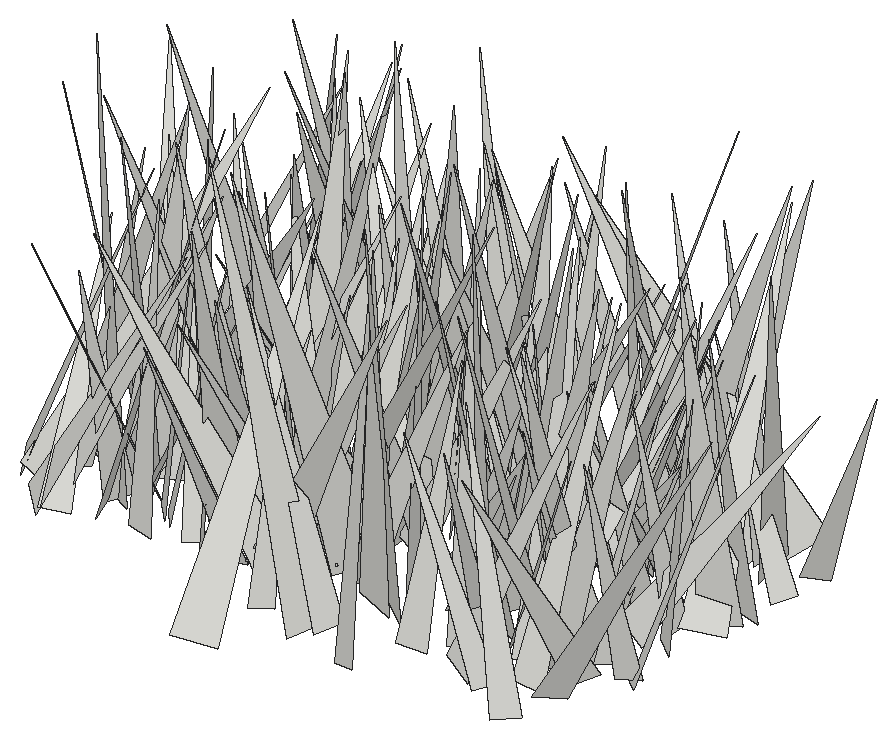
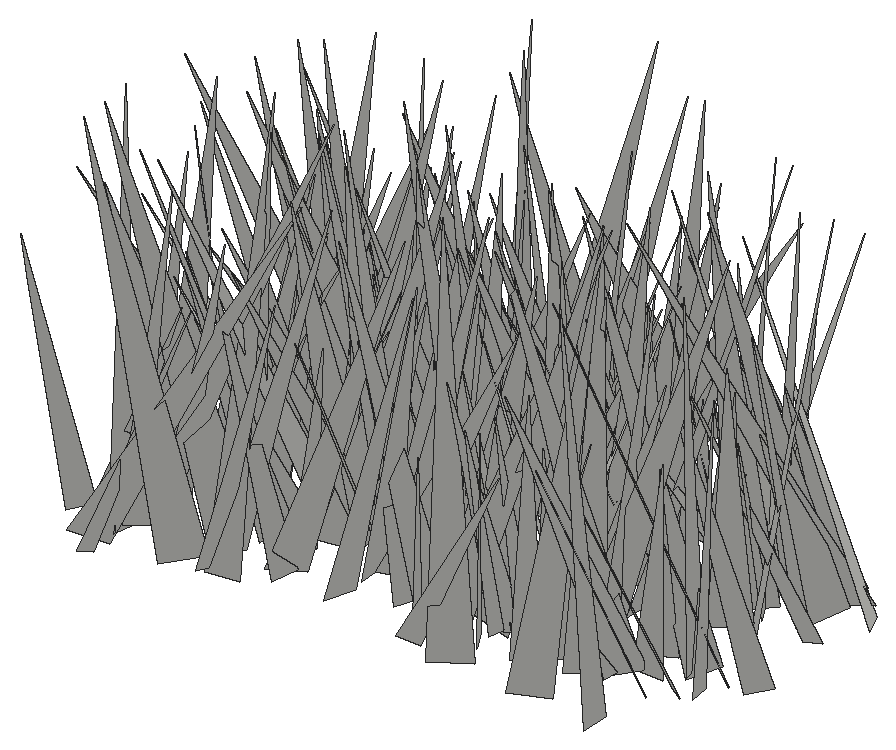
# SketchUp Ruby script. Lengths in inches.
U = 1.inch
M = Sketchup.active_model
def pt(a) = Geom::Point3d.new(a.map { |v| v * U })
def face(e, loops, mat)
  f = e.add_face(loops[0].map { |a| pt(a) })
  loops[1..].each { |l| e.add_face(l.map { |a| pt(a) }).erase! }
  f.material = f.back_material = mat if mat
  f
end
# faces: each face lists its corners as indices into pts; further lists are holes
def faces(e, pts, list, mat = nil) = list.each { |f| face(e, (f[0].is_a?(Array) ? f : [f]).map { |l| l.map { |i| pts[i] } }, mat) }
# xy, xz, yz: faces in a plane at the given z, y or x. An outline is a flat list of corners, or four numbers for a rectangle; further outlines are holes
def ring(l) = l.size == 4 ? [[l[0], l[1]], [l[2], l[1]], [l[2], l[3]], [l[0], l[3]]] : l.each_slice(2).to_a
def flat(e, list, mat, &to3) = list.each { |f| face(e, (f[0].is_a?(Array) ? f : [f]).map { |l| ring(l).map { |u, v| to3.(u, v) } }, mat) }
def xy(e, z, list, mat = nil) = flat(e, list, mat) { |x, y| [x, y, z] }
def xz(e, y, list, mat = nil) = flat(e, list, mat) { |x, z| [x, y, z] }
def yz(e, x, list, mat = nil) = flat(e, list, mat) { |y, z| [x, y, z] }
def lines(e, pts, list) = list.each { |a, b| e.add_line(pt(pts[a]), pt(pts[b])) }
# prism: a flat outline (further loops are holes) pulled along v
def prism(e, loops, v, mat = nil)
  f = face(e, loops, mat); d = Geom::Vector3d.new(v.map { |x| x * U })
  f.pushpull(f.normal.samedirection?(d) ? d.length : -d.length)
end
def box(e, o, s, mat = nil) = prism(e, [[o, [o[0] + s[0], o[1], o[2]], [o[0] + s[0], o[1] + s[1], o[2]], [o[0], o[1] + s[1], o[2]]]], [0, 0, s[2]], mat)
def at(x, y, z, deg = 0) = Geom::Transformation.translation(pt([x, y, z])) * Geom::Transformation.rotation(ORIGIN, Z_AXIS, deg.degrees)
def axes(o, x, y, z) = Geom::Transformation.new([*x, 0, *y, 0, *z, 0, *pt(o).to_a, 1])
def part(name) = M.definitions.add(name)
# library, detail: a bought-in or finely detailed component or shape, given as its bounding box
def library(name, o, s) = part(name).tap { |d| box(d.entities, o, s) }
def detail(e, o, s) = box(e.add_group.entities, o, s)
def put(e, d, t, mat = nil) = e.add_instance(d, t).tap { |i| i.material = mat if mat }
def group(e, t, mat = nil) = e.add_group.tap { |g| g.transformation = t; g.material = mat if mat }.entities
root = M.entities
c1 = part("fur_instance\#9")
p = [[0.8125,0,1.79],[0.67,-0.02,1.48],[0,-0.11,0],[0,0.11,0]]
faces(c1.entities,p,[[0,1,2,3]])
put(root,c1,axes([540.17,98.5,-21.86],[-8.02945,1.44749,0.94959],[1.4539,8.08421,-0.0293],[0.93976,-0.13944,8.15883]))
put(root,c1,axes([546.05,100.68,-21.86],[0.47232,-5.02453,0.37853],[-5.03579,-0.45765,0.20889],[0.17316,0.39615,5.04235]))
put(root,c1,axes([548.83,97.91,-21.86],[-1.63602,4.97918,0.62205],[4.87533,1.42244,1.43652],[-1.18757,-1.0199,5.04036]))
put(root,c1,axes([549.24,101.43,-21.86],[2.87484,-4.36178,0.57915],[-3.91954,-2.85297,-2.03053],[-1.99945,-0.67874,4.81319]))
put(root,c1,axes([537.79,95.55,-21.86],[-4.59589,5.78444,0.11594],[5.4804,4.40003,-2.28044],[1.8543,1.33244,7.02721]))
put(root,c1,axes([547.22,98.81,-21.66],[-1.85647,3.95367,0.8299],[3.82368,1.42492,1.76516],[-1.30372,-1.4508,3.99527]))
put(root,c1,axes([542.79,97.02,-21.66],[2.80201,6.02167,1.40008],[5.6342,-3.12002,2.14317],[-2.54489,-0.27744,6.28638]))
put(root,c1,axes([535.59,100.51,-21.86],[-0.33962,-4.53633,0.58104],[-4.49375,0.22275,-0.88758],[-0.84975,0.63509,4.46159]))
put(root,c1,axes([536.97,100.43,-21.66],[3.33833,-6.51025,0.54896],[-6.14625,-2.92038,2.74304],[2.21549,1.70799,6.78259]))
put(root,c1,axes([537.54,100.35,-21.66],[-4.43221,4.72995,1.58971],[4.78005,3.41433,3.16821],[-1.43205,-3.24253,5.65503]))
put(root,c1,axes([534.4,101.84,-21.86],[6.58115,-3.41587,1.26301],[-3.10443,-6.62563,-1.74311],[-1.90417,-1.00387,7.20703]))
put(root,c1,axes([540.65,98.98,-21.86],[-5.80532,1.01557,0.17125],[1.00882,5.80466,-0.22508],[0.20737,0.19232,5.88918]))
put(root,c1,axes([530.66,102.54,-21.86],[-3.25593,-5.45811,0.05054],[-5.36708,3.21208,1.12765],[0.99394,-0.53501,6.25464]))
put(root,c1,axes([541.5,101.19,-21.86],[-3.95013,-6.45103,2.53754],[-6.55598,4.42551,1.04517],[2.25256,1.56763,7.49179]))
put(root,c1,axes([545.56,99.47,-21.86],[2.52048,5.79703,1.2985],[5.75928,-2.03853,-2.07834],[1.45681,-1.97061,5.96983]))
put(root,c1,axes([539.12,102.41,-21.66],[5.28612,-6.00356,2.19792],[-5.60526,-5.72373,-2.15328],[-3.07484,0.113,7.70384]))
put(root,c1,axes([527.83,99.65,-21.86],[4.10268,4.53992,0.30052],[4.35228,-3.79801,-2.04106],[1.3262,-1.58032,5.76861]))
put(root,c1,axes([534.44,100.1,-21.86],[-2.65775,-2.55388,1.91088],[-2.80676,3.05414,0.17806],[1.51521,1.17784,3.68161]))
put(root,c1,axes([536.71,102.91,-21.66],[-4.92711,-3.11526,0.5387],[-2.69685,4.66208,2.29422],[1.64986,-1.68274,5.3589]))
put(root,c1,axes([540.82,101.11,-21.86],[-1.6159,-6.90986,2.38073],[-7.13771,2.01606,1.00679],[1.57067,2.05292,7.0245]))
put(root,c1,axes([538.32,98.36,-21.66],[-4.43133,1.84787,0.51045],[1.62369,4.30117,-1.47494],[1.01922,1.18203,4.56901]))
put(root,c1,axes([529.97,101.49,-21.86],[3.7662,-3.06911,1.25827],[-2.92554,-3.97067,-0.92842],[-1.56328,0.03677,4.76883]))
put(root,c1,axes([543.54,99.63,-21.86],[-0.63443,5.02312,1.44392],[5.17666,0.80438,-0.52377],[0.72032,-1.3566,5.03586]))
put(root,c1,axes([549.0625,99.86,-21.86],[5.8068,-2.41673,0.19711],[-2.36119,-5.5195,1.88633],[0.55156,1.81463,6.0001]))
put(root,c1,axes([539.56,99.71,-21.66],[-6.70794,-1.60484,0.19836],[-1.59675,6.44001,-1.8942],[-0.25542,1.88735,6.63204]))
put(root,c1,axes([528.1875,100.27,-21.86],[3.52755,5.08967,0.59914],[4.90233,-3.13928,-2.19532],[1.49362,-1.71683,5.79042]))
put(root,c1,axes([531.9,100.13,-21.86],[1.56528,5.39191,1.82425],[5.61252,-1.77733,0.43748],[-0.9488,-1.61836,5.59744]))
put(root,c1,axes([547.9375,101.375,-21.86],[-2.90009,-5.61636,1.60668],[-5.82709,2.65472,-1.23809],[-0.41218,1.98605,6.19848]))
put(root,c1,axes([545.92,101.91,-21.86],[4.89387,1.35478,0.49174],[1.44124,-4.60961,-1.64362],[-0.00784,-1.71558,4.80457]))
put(root,c1,axes([538.1875,100.87,-21.86],[3.85266,4.81198,3.39076],[5.17881,-4.69725,0.78179],[-2.79863,-2.06788,6.11449]))
put(root,c1,axes([533.92,103.66,-21.66],[4.85347,-3.26157,0.26621],[-3.0891,-4.72355,-1.55255],[-1.07988,-1.1468,5.6377]))
put(root,c1,axes([547.32,103.57,-21.86],[3.26606,-6.16963,0.62937],[-6.14796,-3.31446,-0.58694],[-0.81426,0.27855,6.95607]))
put(root,c1,axes([530.28,103.02,-21.86],[-6.05203,-3.65216,2.90127],[-3.20675,6.70926,1.75646],[3.38709,-0.1736,6.84691]))
put(root,c1,axes([534.875,103.26,-21.86],[-3.8372,-2.33717,0.79383],[-2.01321,3.81242,1.493],[1.42812,-0.90538,4.23762]))
put(root,c1,axes([545.36,101.22,-21.86],[-6.66859,-2.01923,2.71074],[-2.32845,7.09045,-0.44648],[2.45024,1.24248,6.95328]))
put(root,c1,axes([550.3,102.4,-21.86],[1.30026,-4.12004,1.09762],[-4.18224,-1.45572,-0.50983],[-0.82967,0.8811,4.29016]))
put(root,c1,axes([528.86,99.52,-21.86],[-2.17484,4.53028,0.06229],[4.50087,2.16823,-0.54601],[0.51907,0.1805,4.99552]))
put(root,c1,axes([525.98,101.5,-21.86],[5.98281,3.47845,0.55141],[3.51313,-5.81778,-1.41742],[0.2481,-1.50052,6.77381]))
put(root,c1,axes([529.96,100.625,-21.86],[6.78168,2.91502,1.19431],[2.8839,-6.88568,0.43057],[-1.26762,-0.07012,7.36906]))
put(root,c1,axes([547.12,103.48,-21.86],[1.17594,-4.92519,0.34785],[-4.93492,-1.18388,-0.07952],[-0.1583,0.31979,5.06301]))
put(root,c1,axes([531.69,101.62,-21.86],[3.10895,3.01642,1.49943],[3.22004,-3.26039,-0.11754],[-0.98914,-1.13301,4.33019]))
put(root,c1,axes([543.23,102.45,-21.86],[2.68666,-2.71893,0.01615],[-2.65256,-2.616,0.85524],[0.59729,0.61233,3.72549]))
put(root,c1,axes([545.07,101.74,-21.86],[3.30994,1.56111,0.94089],[1.62723,-3.40964,-0.0672],[-0.82125,-0.46405,3.659]))
put(root,c1,axes([532.09,101.39,-21.86],[3.54809,3.00738,1.07129],[3.07779,-3.64774,0.04651],[-0.84804,-0.65624,4.65093]))
put(root,c1,axes([534.17,102.42,-21.86],[2.86459,-3.18276,1.27512],[-3.34476,-2.95943,0.1272],[-0.754,1.03614,4.28015]))
put(root,c1,axes([545.59,102.18,-21.86],[-3.32572,-4.76152,1.64129],[-5.0351,3.09772,-1.21581],[-0.11678,2.03921,5.67929]))
put(root,c1,axes([533.67,100.68,-21.86],[-0.67642,4.08917,0.12939],[3.98053,0.62749,0.97839],[-0.94522,-0.2838,4.0276]))
put(root,c1,axes([536.375,102.09,-21.66],[2.73482,-5.11249,1.4467],[-5.08402,-2.04521,2.38319],[1.54377,2.32148,5.28557]))
put(root,c1,axes([529.6,102.18,-21.86],[3.65064,-1.60023,0.53489],[-1.66152,-3.63138,0.47591],[-0.29361,0.65299,3.95745]))
put(root,c1,axes([534.9375,101.64,-21.86],[0.16923,4.07191,1.2027],[4.12697,0.12503,-1.00402],[0.99752,-1.2081,3.94982]))
put(root,c1,axes([547.32,102.4,-21.86],[0.56131,-6.10589,2.64479],[-6.41112,0.21442,1.85565],[1.78167,2.69518,5.8441]))
put(root,c1,axes([530.09,101.33,-21.86],[3.6249,6.4726,3.15784],[6.5149,-4.45394,1.65071],[-3.06961,-1.8095,7.23254]))
put(root,c1,axes([539.4,102.28,-21.66],[-0.77235,4.89048,2.70767],[4.92537,1.88806,-2.00519],[2.64368,-2.08884,4.52687]))
put(root,c1,axes([548.04,99.98,-21.86],[0.77683,6.56918,0.32302],[6.56801,-0.79193,0.30978],[-0.34589,-0.28401,6.60769]))
put(root,c1,axes([549.08,102.7,-21.86],[-1.11932,5.12608,2.18052],[5.30702,0.30525,2.00664],[-1.6932,-2.43194,4.84799]))
put(root,c1,axes([527.42,102.07,-21.86],[6.77248,-2.83159,1.61361],[-3.13932,-6.6674,1.47599],[-0.87537,2.00399,7.19067]))
put(root,c1,axes([529.65,103.11,-21.86],[5.01911,-5.50348,2.14134],[-5.83765,-5.04831,0.7082],[-0.89193,2.07156,7.41473]))
put(root,c1,axes([533.05,104.28,-21.66],[-6.0404,2.2493,3.21945],[3.13358,6.3206,1.46334],[2.36747,-2.62704,6.2773]))
put(root,c1,axes([532.48,105.58,-21.86],[-7.65526,-2.65251,1.50577],[-2.23878,7.64939,2.09305],[2.07148,-1.53532,7.82675]))
put(root,c1,axes([528.44,104.65,-21.86],[-5.36571,-5.00333,1.81378],[-4.95811,5.63559,0.87824],[1.93398,0.5664,7.28374]))
put(root,c1,axes([537.32,102.59,-21.86],[7.55011,-1.58138,0.22082],[-1.59514,-7.42262,1.38345],[0.0711,1.39915,7.58887]))
put(root,c1,axes([547.3125,101.26,-21.66],[-5.92088,3.75972,1.43779],[3.50525,6.07307,-1.44586],[1.97886,0.49178,6.86307]))
put(root,c1,axes([527.1875,100.85,-21.86],[0.81957,8.13408,0.73803],[7.68253,-0.51597,-2.84467],[2.77248,-0.97476,7.66439]))
put(root,c1,axes([540.71,104.28,-21.66],[-1.01411,-6.0227,1.51425],[-5.97973,0.53295,-1.88497],[-1.67593,1.7428,5.80932]))
put(root,c1,axes([544.68,104,-21.86],[7.05562,-2.47543,1.6862],[-2.53392,-7.23407,-0.01726],[-1.59697,0.54154,7.47725]))
put(root,c1,axes([544.84,104.61,-21.86],[2.44609,-6.94499,1.47158],[-6.99231,-2.08787,1.76924],[1.22722,1.94671,7.14745]))
put(root,c1,axes([544.79,100.73,-21.86],[1.27817,7.72916,0.81529],[7.27012,-1.48113,2.64386],[-2.74773,-0.32349,7.37453]))
put(root,c1,axes([541.76,101.9,-21.86],[-6.21182,-1.68937,2.27799],[-2.42044,6.01654,-2.13837],[1.47806,2.75267,6.07191]))
put(root,c1,axes([536.11,106.24,-21.66],[3.38656,-3.48151,1.0277],[-2.77448,-3.38882,-2.33752],[-2.3408,-1.02022,4.25743]))
put(root,c1,axes([527.29,103.43,-21.86],[2.3418,4.95634,1.60959],[5.19702,-2.35112,-0.32146],[-0.38351,-1.59595,5.4723]))
put(root,c1,axes([533.44,105.8125,-21.86],[5.68928,-3.36377,1.44998],[-3.11585,-5.85243,-1.35122],[-1.92583,-0.46842,6.46971]))
put(root,c1,axes([539.49,101.8125,-21.86],[5.41894,2.39891,1.8987],[1.67708,-5.5593,2.23748],[-2.55876,1.4367,5.48756]))
put(root,c1,axes([546.1,102.71,-21.86],[2.83544,5.2975,1.05869],[5.3487,-2.92083,0.29014],[-0.75876,-0.79328,6.00159]))
put(root,c1,axes([530.45,102.22,-21.86],[3.83996,1.68055,0.1423],[1.49178,-3.54944,1.66307],[-0.78682,1.47206,3.84756]))
put(root,c1,axes([538.6,102.56,-21.86],[-1.26821,6.79621,1.34265],[6.86908,1.41065,-0.65215],[0.89826,-1.19212,6.8827]))
put(root,c1,axes([548.79,102.11,-21.86],[2.63197,4.07891,0.20518],[3.86496,-2.5665,1.44292],[-1.31973,0.61842,4.63495]))
put(root,c1,axes([530.49,103.48,-21.86],[-1.05429,4.67357,0.99792],[4.75005,0.91265,0.74413],[-0.52453,-1.12891,4.73287]))
put(root,c1,axes([529.37,102.875,-21.86],[3.31155,2.43431,1.59522],[1.82743,-3.61986,1.73033],[-2.2652,0.63849,3.72802]))
put(root,c1,axes([538.84,102.32,-21.66],[-5.03448,1.97141,0.87824],[1.57247,4.87743,-1.93439],[1.47821,1.52579,5.04882]))
put(root,c1,axes([526.76,103.66,-21.86],[1.36791,4.73736,0.76135],[4.55305,-1.0318,-1.76027],[1.51392,-1.17738,4.60599]))
put(root,c1,axes([544.23,103.75,-21.86],[3.72107,-3.56028,1.90501],[-4.03778,-3.30047,1.71878],[-0.03061,2.5656,4.85467]))
put(root,c1,axes([545.96,104.21,-21.86],[-4.56501,-1.69942,1.47091],[-1.97129,4.62695,-0.77219],[1.07964,1.26263,4.80947]))
put(root,c1,axes([541.9,104.51,-21.66],[6.07863,-4.42165,0.21276],[-4.21796,-5.67554,2.55792],[1.3435,2.18706,7.06807]))
put(root,c1,axes([541.34,105.34,-21.86],[1.54528,-3.8993,0.59524],[-3.77652,-1.27799,1.43226],[1.13873,1.05307,3.94222]))
put(root,c1,axes([550.66,102.11,-21.86],[3.88995,3.95886,0.07672],[3.75671,-3.72392,1.68217],[-1.25122,1.12695,5.2891]))
put(root,c1,axes([538.89,104.78,-21.86],[7.17764,0.6661,2.04171],[0.73913,-7.45363,-0.1667],[-2.01642,-0.36113,7.20655]))
put(root,c1,axes([539.53,104.68,-21.86],[1.43912,5.66343,2.07225],[5.60003,-0.46439,-2.61988],[2.23794,-2.47985,5.22319]))
put(root,c1,axes([547.0625,105.83,-21.86],[-0.84306,-4.44176,0.86686],[-4.52258,0.85891,0.00263],[0.16427,0.85115,4.52106]))
put(root,c1,axes([546.3125,102.7,-21.86],[-0.54715,4.89077,0.10405],[4.53126,0.54616,-1.84371],[1.84341,0.10915,4.56287]))
put(root,c1,axes([548.36,105.83,-21.86],[0.08099,-5.17118,1.20761],[-5.27072,-0.22549,-0.61212],[-0.64729,1.18913,5.13546]))
put(root,c1,axes([535.25,103.83,-21.86],[3.15167,2.15202,0.19961],[2.1362,-3.1554,0.29004],[-0.32814,0.12762,3.80527]))
put(root,c1,axes([540.6,107.68,-21.86],[-2.04467,-7.63412,0.65301],[-7.56547,2.11851,1.07815],[1.21235,0.345,7.82931]))
put(root,c1,axes([544.49,106.01,-21.86],[-1.50167,-7.67594,2.08534],[-7.92089,1.24921,-1.10571],[-0.72669,2.24569,7.7429]))
put(root,c1,axes([534.42,107.93,-21.86],[-4.33714,-4.09832,0.0827],[-3.81397,4.0787,2.10515],[1.50223,-1.4771,5.58349]))
put(root,c1,axes([539.06,103.17,-21.66],[-5.01986,0.40192,1.5189],[-0.17545,4.90978,-1.87904],[1.56135,1.84392,4.67223]))
put(root,c1,axes([535.88,104.28,-21.86],[-4.18107,4.06515,1.12452],[4.17237,4.21812,0.26475],[0.61747,-0.97641,5.82552]))
put(root,c1,axes([549.51,105.85,-21.86],[-4.17455,0.44699,1.70239],[0.80041,4.38471,0.81146],[1.56757,-1.04848,4.11925]))
put(root,c1,axes([546.54,105.26,-21.86],[-3.00148,-2.27694,0.1564],[-2.20162,2.82047,-1.1898],[-0.60148,1.03841,3.57459]))
put(root,c1,axes([539.78,106.43,-21.66],[4.17117,1.8451,1.43695],[2.27213,-3.89306,-1.59669],[-0.55375,-2.07548,4.27243]))
put(root,c1,axes([545.25,105.64,-21.86],[6.75875,-1.16964,0.00047],[-1.16859,-6.75255,0.29358],[0.0496,0.28936,6.85293]))
put(root,c1,axes([534.52,105.68,-21.86],[2.08402,3.38406,1.47593],[3.68931,-1.84524,-0.97848],[0.13865,-1.76538,3.85196]))
put(root,c1,axes([543.46,105.39,-21.86],[-2.68831,3.38264,1.06218],[3.54497,2.54168,0.8778],[-0.06058,-1.37662,4.23069]))
put(root,c1,axes([533.1,103.67,-21.86],[2.76171,5.55128,0.00194],[5.48471,-2.72826,-0.95829],[0.85713,-0.42855,6.1258]))
put(root,c1,axes([549.92,104.74,-21.86],[3.73887,4.62596,1.90486],[4.75099,-4.02818,0.45718],[-1.5672,-1.17533,5.9304]))
put(root,c1,axes([528.01,107.7,-21.66],[1.13503,-7.67663,0.6742],[-6.50823,-0.58999,4.2389],[4.12651,1.18099,6.50005]))
put(root,c1,axes([530.26,104.49,-21.86],[-1.29816,5.29172,0.79515],[5.27739,1.13069,1.0911],[-0.88529,-1.01932,5.33826]))
put(root,c1,axes([538.06,106.75,-21.86],[-0.11111,-7.60969,2.49454],[-7.52897,0.94928,2.56048],[2.72852,2.30953,7.16685]))
put(root,c1,axes([542.48,108.47,-21.66],[3.73251,-5.71066,0.85994],[-5.41751,-3.81707,-1.83396],[-2.00044,-0.31799,6.57114]))
put(root,c1,axes([548.4,104.86,-21.86],[1.31269,5.55847,0.82299],[4.82858,-0.68361,-3.08457],[2.8738,-1.39037,4.80678]))
put(root,c1,axes([545.89,104.03,-21.86],[-1.09311,5.26549,0.63584],[5.05113,1.23151,-1.51458],[1.61731,-0.28736,5.16007]))
put(root,c1,axes([534.16,103.17,-21.66],[3.4696,4.95294,0.18512],[4.68916,-3.35343,1.83583],[-1.60551,0.90933,5.7619]))
put(root,c1,axes([548.71,107.12,-21.86],[-1.81586,-4.37557,0.34615],[-4.20637,1.62778,-1.48984],[-1.25376,0.87607,4.49704]))
put(root,c1,axes([550.4,107.01,-21.86],[-2.64442,5.36733,3.49605],[6.32318,2.79183,0.49668],[1.02376,-3.3795,5.96276]))
put(root,c1,axes([534.57,105.31,-21.86],[-5.26533,5.42334,2.66225],[5.51698,5.75546,-0.81326],[2.46233,-1.29842,7.51498]))
put(root,c1,axes([535.9,102.54,-21.66],[7.29611,1.84526,3.54482],[-0.04664,-7.33917,3.91643],[-3.99607,3.45479,6.4265]))
put(root,c1,axes([543.5,105.21,-21.86],[-5.91196,3.62871,1.99788],[3.48429,6.23911,-1.02156],[2.24027,-0.12769,6.86114]))
put(root,c1,axes([529.49,104.51,-21.86],[-4.42637,5.44798,0.10976],[5.44745,4.42761,-0.08267],[0.13338,-0.03304,7.019]))
put(root,c1,axes([543.73,107.28,-21.86],[-3.71371,1.13934,1.58672],[1.47505,3.87017,0.67337],[1.28063,-1.15373,3.82574]))
put(root,c1,axes([541.4,106.7,-21.86],[7.16515,0.1083,1.44204],[0.09788,-7.3087,0.06254],[-1.44279,0.042,7.1657]))
put(root,c1,axes([547.18,106.04,-21.86],[-1.55107,4.41542,0.77186],[4.34501,1.28043,1.40671],[-1.10114,-1.16708,4.46351]))
put(root,c1,axes([534.38,105.05,-21.66],[-2.83058,6.09964,1.95872],[5.76034,3.3604,-2.14023],[2.80369,-0.74599,6.37473]))
put(root,c1,axes([526.08,107.27,-21.86],[2.085,-4.49657,0.98747],[-4.39792,-1.62495,1.88661],[1.36107,1.63764,4.58334]))
put(root,c1,axes([533.18,107.03,-21.86],[-1.13244,4.66111,1.93868],[4.91983,0.57378,1.4943],[-1.13125,-2.17064,4.55801]))
put(root,c1,axes([550.67,108.01,-21.86],[-1.20745,-5.31811,1.49773],[-5.50418,1.29079,0.14593],[0.47907,1.42653,5.45151]))
put(root,c1,axes([531.26,109.77,-21.86],[6.38115,-3.67921,0.2036],[-3.55943,-6.25987,-1.56256],[-0.95316,-1.25481,7.1982]))
put(root,c1,axes([528.67,107.33,-21.86],[-5.78196,-1.74059,3.08913],[-1.82129,6.52793,0.26926],[3.04225,0.59997,6.03227]))
put(root,c1,axes([538.53,106.22,-21.86],[0.66704,7.88186,2.68055],[8.14998,-1.16705,1.40349],[-1.69907,-2.50365,7.78452]))
put(root,c1,axes([547.65,105.19,-21.86],[3.29969,3.36632,0.10349],[3.25213,-3.22241,1.12716],[-0.87548,0.71745,4.57707]))
put(root,c1,axes([534.98,106.17,-21.86],[1.28068,6.67783,2.12971],[6.86225,-1.63556,1.00185],[-1.42781,-1.87102,6.72532]))
put(root,c1,axes([531.0625,108.85,-21.66],[5.81845,-0.62274,2.18855],[-0.03101,-6.03017,-1.6334],[-2.27522,-1.51035,5.61909]))
put(root,c1,axes([538.79,105.92,-21.86],[-4.59485,5.55244,0.46156],[5.5505,4.50971,1.00485],[-0.48434,-0.99407,7.1367]))
put(root,c1,axes([532.07,108.39,-21.86],[-0.48012,-7.554,2.16495],[-7.6037,-0.10085,-2.03814],[-1.98335,2.21526,7.28968]))
put(root,c1,axes([538.05,109.13,-21.86],[4.30794,-3.29071,0.86204],[-3.07513,-4.36194,-1.28347],[-1.45447,-0.52435,5.26686]))
put(root,c1,axes([536.04,105.44,-21.86],[3.8094,4.08661,1.06154],[3.80016,-3.94157,1.53675],[-1.84012,0.32005,5.37125]))
put(root,c1,axes([529.87,107.32,-21.86],[1.56835,-2.82264,1.69633],[-3.20586,-1.73838,0.07137],[-0.75322,1.52161,3.2283]))
put(root,c1,axes([547.625,106.17,-21.86],[3.89268,2.82638,0.90518],[2.67493,-3.98806,0.94914],[-1.28551,0.26015,4.71599]))
put(root,c1,axes([544.87,107.58,-21.86],[2.65844,-2.5721,0.0216],[-2.2994,-2.3625,1.67773],[1.15278,1.21916,3.2967]))
put(root,c1,axes([536.25,108.9,-21.86],[4.56733,-2.95407,1.62637],[-2.80415,-4.84794,-0.93072],[-1.87305,0.05455,5.35918]))
put(root,c1,axes([527.51,108.58,-21.86],[-4.30625,-1.78107,2.16646],[-1.55574,4.81995,0.87021],[2.33354,-0.07334,4.57807]))
put(root,c1,axes([540.49,106.95,-21.86],[-1.13275,3.97734,1.11963],[3.98013,1.3621,-0.81189],[1.10966,-0.82546,4.05502]))
put(root,c1,axes([544.625,105.33,-21.86],[-6.84761,2.51212,1.52779],[1.98246,6.80446,-2.30302],[2.17135,1.70976,6.92074]))
put(root,c1,axes([545.39,105.92,-21.66],[-6.80362,-1.51626,0.05987],[-1.39466,6.13985,-2.9915],[-0.59797,2.93174,6.29597]))
put(root,c1,axes([532.43,109.5625,-21.86],[7.09602,-3.54407,1.49132],[-3.45875,-7.25092,-0.77408],[-1.67974,-0.04148,7.89397]))
put(root,c1,axes([540.1875,107.78,-21.86],[-7.39383,1.79038,1.19471],[1.82356,7.48136,0.07416],[1.14343,-0.35412,7.60715]))
put(root,c1,axes([534.71,108.91,-21.86],[4.32257,0.5968,0.21737],[0.63053,-4.21214,-0.97382],[-0.07654,-0.99484,4.25352]))
put(root,c1,axes([545.97,108.55,-21.86],[2.87262,5.81566,3.24646],[6.49078,-3.23727,0.05584],[-1.49368,-2.88298,6.48619]))
put(root,c1,axes([538.4,109.93,-21.66],[7.85727,-0.11013,0.63762],[0.0287,-7.70188,-1.68396],[-0.64642,-1.6806,7.67549]))
put(root,c1,axes([536.65,110.16,-21.86],[-1.86183,-7.54983,1.10161],[-7.50699,1.61006,-1.65309],[-1.3633,1.44488,7.59827]))
put(root,c1,axes([527.13,107.69,-21.66],[4.92095,5.18553,0.33695],[5.09859,-4.72846,-1.69263],[1.00379,-1.4039,6.94554]))
put(root,c1,axes([541.93,107.28,-21.66],[5.39304,-0.33096,0.39775],[-0.43435,-5.15892,1.59671],[-0.28121,1.6213,5.16187]))
put(root,c1,axes([535.75,109.24,-21.86],[-0.98581,-7.65367,2.64082],[-7.9173,0.35473,-1.92744],[-1.69382,2.79641,7.47232]))
put(root,c1,axes([534.04,108.98,-21.86],[-3.00946,-2.45302,0.73779],[-2.54129,3.00205,-0.38468],[0.32167,0.76736,3.86344]))
put(root,c1,axes([543.53,109,-21.86],[1.53479,-3.08573,1.52348],[-3.30012,-1.79268,-0.30636],[-0.97569,1.2095,3.43271]))
put(root,c1,axes([530.46,108.9,-21.86],[7.76844,-0.71206,0.72464],[-0.74639,-7.79129,0.34557],[-0.68922,0.41169,7.79335]))
put(root,c1,axes([539.83,108.93,-21.66],[-4.53112,4.00144,0.54603],[3.94801,4.21612,1.86503],[-0.85024,-1.74745,5.75015]))
put(root,c1,axes([549.41,110.99,-21.86],[7.02659,-0.33713,1.59],[0.09653,-6.95626,-1.90152],[-1.62247,-1.87389,6.7728]))
put(root,c1,axes([533.49,109.875,-21.86],[1.4619,-3.63585,0.57448],[-3.60479,-1.28901,1.01518],[0.74496,0.89757,3.78497]))
put(root,c1,axes([544.45,108.55,-21.86],[3.65176,6.04586,1.11201],[6.02251,-3.25936,-2.05677],[1.23222,-1.98709,6.75703]))
put(root,c1,axes([544.86,109.13,-21.86],[5.19271,0.37939,0.34653],[0.38191,-5.20401,-0.02543],[-0.34375,-0.05067,5.20649]))
put(root,c1,axes([550.23,106.3,-21.86],[-3.4412,6.39637,0.09759],[6.32165,3.41718,-1.06042],[0.97968,0.41743,7.18546]))
put(root,c1,axes([544.52,106.54,-21.86],[7.12213,3.78972,1.00867],[3.4176,-7.02352,2.25704],[-1.92338,1.55314,7.74548]))
put(root,c1,axes([548.55,111.15,-21.86],[-7.92246,2.32052,1.49756],[2.68865,7.5204,2.57051],[0.63138,-2.90715,7.84491]))
put(root,c1,axes([544.36,112.19,-21.86],[-1.3783,-7.92591,0.91068],[-7.76861,1.54372,1.6777],[1.81604,0.58822,7.86798]))
put(root,c1,axes([531.5,112.4,-21.66],[5.49992,-4.64771,0.52674],[-4.40214,-5.41809,-1.84207],[-1.58109,-1.08206,6.96111]))
put(root,c1,axes([529.61,108.62,-21.86],[-1.32199,4.73147,0.88748],[4.77716,1.17578,0.84759],[-0.59431,-1.0737,4.83901]))
put(root,c1,axes([543.03,110.55,-21.86],[-5.87282,3.13064,1.60123],[3.47052,5.66214,1.65846],[0.56601,-2.23474,6.44519]))
put(root,c1,axes([545.16,110.82,-21.86],[-6.41083,1.14128,1.69671],[1.48537,6.43646,1.28286],[1.40536,-1.59673,6.38401]))
put(root,c1,axes([528.1,109.04,-21.86],[2.47782,3.1575,0.0552],[3.13992,-2.45577,-0.47176],[0.33732,-0.3344,3.98583]))
put(root,c1,axes([550.98,109.625,-21.86],[-4.27711,1.68369,0.0136],[1.68167,4.26988,0.26227],[-0.08344,-0.24902,4.58909]))
put(root,c1,axes([537.16,110.07,-21.86],[-0.35143,6.05342,2.99786],[6.31844,1.35633,-1.99808],[2.38924,-2.69649,5.72495]))
put(root,c1,axes([545.96,109.66,-21.86],[6.10397,-4.61293,1.81963],[-4.95361,-5.80478,1.9013],[-0.22786,2.62185,7.41098]))
put(root,c1,axes([533.19,110.43,-21.86],[1.68942,-4.24341,1.91691],[-4.60334,-1.82876,0.00876],[-0.70022,1.78447,4.56734]))
put(root,c1,axes([535.07,109.36,-21.86],[3.50267,-1.34823,2.1537],[-1.97697,-3.75014,0.86764],[-1.59615,1.68627,3.65152]))
put(root,c1,axes([535.07,112.01,-21.86],[3.4393,-6.56896,1.063],[-6.65437,-3.3911,0.57422],[0.02233,1.20797,7.39258]))
put(root,c1,axes([535.25,110.3,-21.86],[3.08289,1.97486,1.70839],[2.08981,-3.45082,0.21788],[-1.56569,-0.71742,3.6547]))
put(root,c1,axes([534.85,109.23,-21.86],[-1.16488,5.07104,1.08343],[5.11451,1.30667,-0.61696],[0.85504,-0.90739,5.16641]))
put(root,c1,axes([542.83,110.86,-21.86],[5.32067,-0.59583,0.38531],[-0.58759,-5.33383,-0.13414],[-0.39777,-0.09079,5.35224]))
put(root,c1,axes([541.11,107.95,-21.86],[2.7978,5.22834,0.27095],[4.99402,-2.75746,1.64099],[-1.57121,0.54549,5.69828]))
put(root,c1,axes([540.66,110.75,-21.86],[-6.00997,1.04438,1.22572],[1.13938,6.10462,0.38513],[1.13796,-0.59647,6.08787]))
put(root,c1,axes([548.47,109.61,-21.86],[-6.22467,1.67352,0.58559],[1.62437,6.23957,-0.56507],[0.71064,0.39649,6.42089]))
put(root,c1,axes([540.51,108.81,-21.66],[-7.44461,1.33123,0.56849],[1.18187,7.30967,-1.63995],[0.83578,1.52121,7.38274]))
put(root,c1,axes([550.85,111.37,-21.86],[3.25053,-3.28963,0.28157],[-3.26975,-3.15258,0.91484],[0.45796,0.84053,4.53329]))
put(root,c1,axes([549.39,112.83,-21.86],[-6.27712,3.42033,1.55819],[3.73626,5.34865,3.31076],[-0.40863,-3.63622,6.33559]))
put(root,c1,axes([548.78,111.51,-21.86],[5.59524,-0.57904,3.08549],[-0.36766,-6.38318,-0.53118],[-3.11775,-0.28642,5.59999]))
put(root,c1,axes([529.125,109.53,-21.86],[2.95968,3.81178,0.17357],[3.80838,-2.96454,0.16477],[-0.23661,-0.0359,4.82309]))
put(root,c1,axes([530.19,108.92,-21.86],[-2.51338,5.74575,1.01303],[5.46798,2.70448,-1.77311],[2.03497,-0.17044,6.01555]))
put(root,c1,axes([528.93,112.21,-21.86],[6.91292,1.02767,1.79019],[1.3308,-7.00178,-1.11957],[-1.57792,-1.40299,6.89863]))
put(root,c1,axes([545.08,111.96,-21.86],[-4.85785,0.78834,1.37895],[1.02249,4.94749,0.77364],[1.21552,-1.0112,4.86021]))
put(root,c1,axes([537.35,110.85,-21.86],[1.49909,3.09185,1.25062],[3.12666,-1.78006,0.6529],[-1.16087,-0.8017,3.3735]))
put(root,c1,axes([548.89,113.62,-21.86],[-4.22388,-0.55824,1.0602],[-0.01996,3.91714,1.98304],[1.19803,-1.90295,3.77099]))
put(root,c1,axes([536.82,112.01,-21.66],[-2.52237,2.99386,0.77548],[2.99232,2.10973,1.58806],[-0.78138,-1.58517,3.57821]))
put(root,c1,axes([546.05,112.12,-21.86],[4.37755,-6.1842,1.75356],[-6.40379,-4.01166,1.83857],[0.55746,2.47882,7.3503]))
